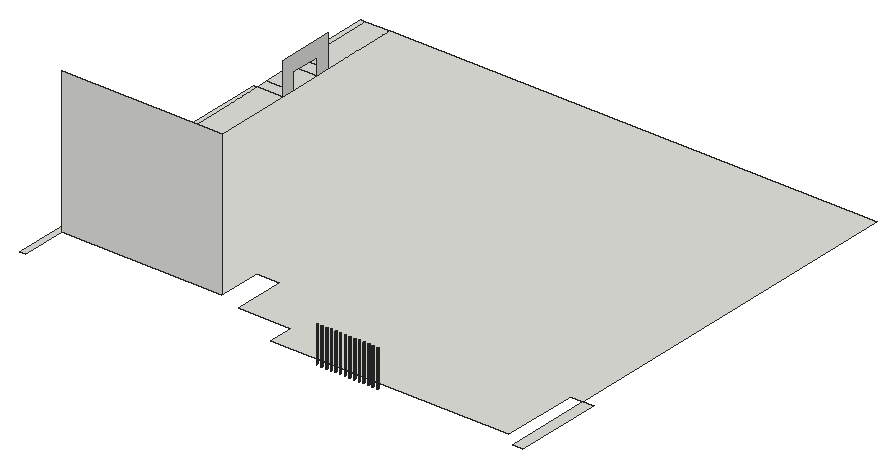
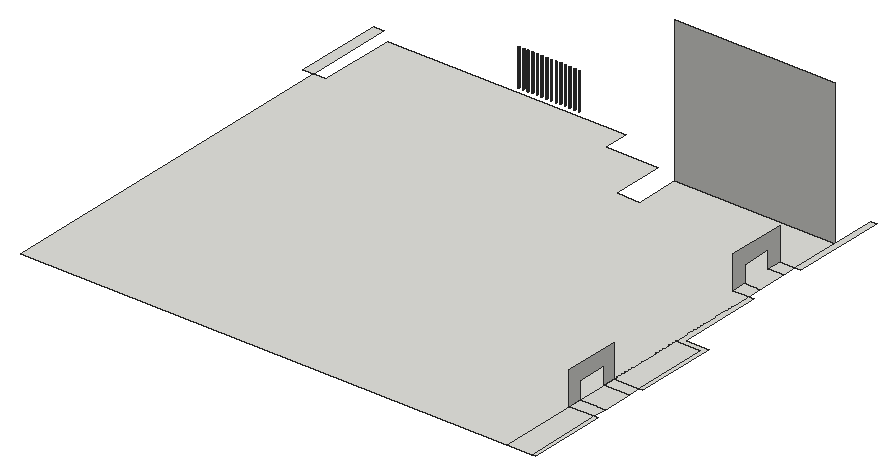
# SketchUp Ruby script. Lengths in inches.
U = 1.inch
M = Sketchup.active_model
def pt(a) = Geom::Point3d.new(a.map { |v| v * U })
def face(e, loops, mat)
  f = e.add_face(loops[0].map { |a| pt(a) })
  loops[1..].each { |l| e.add_face(l.map { |a| pt(a) }).erase! }
  f.material = f.back_material = mat if mat
  f
end
# faces: each face lists its corners as indices into pts; further lists are holes
def faces(e, pts, list, mat = nil) = list.each { |f| face(e, (f[0].is_a?(Array) ? f : [f]).map { |l| l.map { |i| pts[i] } }, mat) }
# xy, xz, yz: faces in a plane at the given z, y or x. An outline is a flat list of corners, or four numbers for a rectangle; further outlines are holes
def ring(l) = l.size == 4 ? [[l[0], l[1]], [l[2], l[1]], [l[2], l[3]], [l[0], l[3]]] : l.each_slice(2).to_a
def flat(e, list, mat, &to3) = list.each { |f| face(e, (f[0].is_a?(Array) ? f : [f]).map { |l| ring(l).map { |u, v| to3.(u, v) } }, mat) }
def xy(e, z, list, mat = nil) = flat(e, list, mat) { |x, y| [x, y, z] }
def xz(e, y, list, mat = nil) = flat(e, list, mat) { |x, z| [x, y, z] }
def yz(e, x, list, mat = nil) = flat(e, list, mat) { |y, z| [x, y, z] }
def lines(e, pts, list) = list.each { |a, b| e.add_line(pt(pts[a]), pt(pts[b])) }
# prism: a flat outline (further loops are holes) pulled along v
def prism(e, loops, v, mat = nil)
  f = face(e, loops, mat); d = Geom::Vector3d.new(v.map { |x| x * U })
  f.pushpull(f.normal.samedirection?(d) ? d.length : -d.length)
end
def box(e, o, s, mat = nil) = prism(e, [[o, [o[0] + s[0], o[1], o[2]], [o[0] + s[0], o[1] + s[1], o[2]], [o[0], o[1] + s[1], o[2]]]], [0, 0, s[2]], mat)
def at(x, y, z, deg = 0) = Geom::Transformation.translation(pt([x, y, z])) * Geom::Transformation.rotation(ORIGIN, Z_AXIS, deg.degrees)
def axes(o, x, y, z) = Geom::Transformation.new([*x, 0, *y, 0, *z, 0, *pt(o).to_a, 1])
def part(name) = M.definitions.add(name)
# library, detail: a bought-in or finely detailed component or shape, given as its bounding box
def library(name, o, s) = part(name).tap { |d| box(d.entities, o, s) }
def detail(e, o, s) = box(e.add_group.entities, o, s)
def put(e, d, t, mat = nil) = e.add_instance(d, t).tap { |i| i.material = mat if mat }
def group(e, t, mat = nil) = e.add_group.tap { |g| g.transformation = t; g.material = mat if mat }.entities
root = M.entities
M.materials.add("Generic\#2").color = [186, 186, 186]
xy(root,1024.6875,[[41,124.5,48.5,249],[690.4375,124.5,703.6875,241.25],[359.25,139.4375,673.48,139.4375,673.48,241.25,690.4375,241.25,690.4375,724.5,48.5,724.5,48.5,326.1875,69,326.1875,69,306.87,48.5,306.87,48.5,268.32,69,268.32,69,249,48.5,249,48.5,183.25,259.3125,183.25,259.3125,241.25,290.4375,241.25,290.4375,172.5,359.25,172.5],[48.5,249,69,268.32],[48.5,306.87,69,326.1875],
  [41,326.1875,48.5,326.1875,48.5,446.1875,15.3125,446.1875,15.3125,547.73,10.5,547.73,10.5,438.6875,41,438.6875],[15.3125,446.1875,48.5,547.73],[15.3125,547.73,48.5,563.94],[15.3125,563.94,48.5,603.53],[15.3125,603.53,48.5,621.86],
  [10.5,621.86,15.3125,724.5],[15.3125,621.86,48.5,724.5]])
xz(root,183.25,[[48.5,1024.6875,259.3125,1214.9375]])
yz(root,48.5,[[547.73,1024.6875,563.94,1024.6875,563.94,1046.8125,603.53,1046.8125,603.53,1024.6875,621.86,1024.6875,621.86,1067.5625,547.73,1067.5625]])
yz(root,69,[[249,1024.6875,268.32,1024.6875,268.32,1046.8125,306.87,1046.8125,306.87,1024.6875,326.1875,1024.6875,326.1875,1067.5625,249,1067.5625]])
p = [[427.76,129.86,1024.6875],[427.96,129.78,1024.6875],[427.96,129.78,1072.38],[427.76,129.86,1072.38],[428.17,129.75,1024.6875],[428.17,129.75,1072.38],
  [428.38,129.78,1024.6875],[428.38,129.78,1072.38],[428.57,129.86,1024.6875],[428.57,129.86,1072.38],[433.82,129.86,1024.6875],[434.02,129.78,1024.6875],
  [434.02,129.78,1072.38],[433.82,129.86,1072.38],[434.23,129.75,1024.6875],[434.23,129.75,1072.38],[434.44,129.78,1024.6875],[434.44,129.78,1072.38],
  [434.64,129.86,1024.6875],[434.64,129.86,1072.38],[439.95,129.86,1024.6875],[440.15,129.78,1024.6875],[440.15,129.78,1072.38],[439.95,129.86,1072.38],
  [440.36,129.75,1024.6875],[440.36,129.75,1072.38],[440.57,129.78,1024.6875],[440.57,129.78,1072.38],[440.76,129.86,1024.6875],[440.76,129.86,1072.38],
  [445.95,129.86,1024.6875],[446.15,129.78,1024.6875],[446.15,129.78,1072.38],[445.95,129.86,1072.38],[446.36,129.75,1024.6875],[446.36,129.75,1072.38],
  [446.57,129.78,1024.6875],[446.57,129.78,1072.38],[446.76,129.86,1024.6875],[446.76,129.86,1072.38],[452.2,129.86,1024.6875],[452.4,129.78,1024.6875],
  [452.4,129.78,1072.38],[452.2,129.86,1072.38],[452.61,129.75,1024.6875],[452.61,129.75,1072.38],[452.82,129.78,1024.6875],[452.82,129.78,1072.38],
  [453.01,129.86,1024.6875],[453.01,129.86,1072.38],[458.14,129.86,1024.6875],[458.33,129.78,1024.6875],[458.33,129.78,1072.38],[458.14,129.86,1072.38],
  [458.54,129.75,1024.6875],[458.54,129.75,1072.38],[458.75,129.78,1024.6875],[458.75,129.78,1072.38],[458.95,129.86,1024.6875],[458.95,129.86,1072.38],
  [464.39,129.86,1024.6875],[464.58,129.78,1024.6875],[464.58,129.78,1072.38],[464.39,129.86,1072.38],[464.79,129.75,1024.6875],[464.79,129.75,1072.38],
  [465,129.78,1024.6875],[465,129.78,1072.38],[465.2,129.86,1024.6875],[465.2,129.86,1072.38],[470.76,129.86,1024.6875],[470.96,129.78,1024.6875],
  [470.96,129.78,1072.38],[470.76,129.86,1072.38],[471.17,129.75,1024.6875],[471.17,129.75,1072.38],[471.38,129.78,1024.6875],[471.38,129.78,1072.38],
  [471.57,129.86,1024.6875],[471.57,129.86,1072.38],[476.76,129.86,1024.6875],[476.96,129.78,1024.6875],[476.96,129.78,1072.38],[476.76,129.86,1072.38],
  [477.17,129.75,1024.6875],[477.17,129.75,1072.38],[477.38,129.78,1024.6875],[477.38,129.78,1072.38],[477.57,129.86,1024.6875],[477.57,129.86,1072.38],
  [482.82,129.86,1024.6875],[483.02,129.78,1024.6875],[483.02,129.78,1072.38],[482.82,129.86,1072.38],[483.23,129.75,1024.6875],[483.23,129.75,1072.38],
  [483.44,129.78,1024.6875],[483.44,129.78,1072.38],[483.64,129.86,1024.6875],[483.64,129.86,1072.38],[489.2,129.86,1024.6875],[489.4,129.78,1024.6875],
  [489.4,129.78,1072.38],[489.2,129.86,1072.38],[489.61,129.75,1024.6875],[489.61,129.75,1072.38],[489.82,129.78,1024.6875],[489.82,129.78,1072.38],
  [490.01,129.86,1024.6875],[490.01,129.86,1072.38],[495.2,129.86,1024.6875],[495.4,129.78,1024.6875],[495.4,129.78,1072.38],[495.2,129.86,1072.38],
  [495.61,129.75,1024.6875],[495.61,129.75,1072.38],[495.82,129.78,1024.6875],[495.82,129.78,1072.38],[496.01,129.86,1024.6875],[496.01,129.86,1072.38],
  [501.2,129.86,1024.6875],[501.4,129.78,1024.6875],[501.4,129.78,1072.38],[501.2,129.86,1072.38],[501.61,129.75,1024.6875],[501.61,129.75,1072.38],
  [501.82,129.78,1024.6875],[501.82,129.78,1072.38],[502.01,129.86,1024.6875],[502.01,129.86,1072.38],[507.2,129.86,1024.6875],[507.4,129.78,1024.6875],
  [507.4,129.78,1072.38],[507.2,129.86,1072.38],[507.61,129.75,1024.6875],[507.61,129.75,1072.38],[507.82,129.78,1024.6875],[507.82,129.78,1072.38],
  [508.01,129.86,1024.6875],[508.01,129.86,1072.38],[427.59,129.99,1024.6875],[427.59,129.99,1072.38],[433.66,129.99,1024.6875],[433.66,129.99,1072.38],
  [434.81,129.99,1024.6875],[434.81,129.99,1072.38],[439.78,129.99,1024.6875],[439.78,129.99,1072.38],[440.93,129.99,1024.6875],[440.93,129.99,1072.38],
  [445.78,129.99,1024.6875],[445.78,129.99,1072.38],[446.93,129.99,1024.6875],[446.93,129.99,1072.38],[452.03,129.99,1024.6875],[452.03,129.99,1072.38],
  [453.18,129.99,1024.6875],[453.18,129.99,1072.38],[457.97,129.99,1024.6875],[457.97,129.99,1072.38],[459.12,129.99,1024.6875],[459.12,129.99,1072.38],
  [464.22,129.99,1024.6875],[464.22,129.99,1072.38],[465.37,129.99,1024.6875],[465.37,129.99,1072.38],[470.59,129.99,1024.6875],[470.59,129.99,1072.38],
  [471.74,129.99,1024.6875],[471.74,129.99,1072.38],[476.59,129.99,1024.6875],[476.59,129.99,1072.38],[477.74,129.99,1024.6875],[477.74,129.99,1072.38],
  [482.66,129.99,1024.6875],[482.66,129.99,1072.38],[483.81,129.99,1024.6875],[483.81,129.99,1072.38],[489.03,129.99,1024.6875],[489.03,129.99,1072.38],
  [490.18,129.99,1024.6875],[490.18,129.99,1072.38],[495.03,129.99,1024.6875],[495.03,129.99,1072.38],[496.18,129.99,1024.6875],[496.18,129.99,1072.38],
  [501.03,129.99,1024.6875],[501.03,129.99,1072.38],[502.18,129.99,1024.6875],[502.18,129.99,1072.38],[507.03,129.99,1024.6875],[507.03,129.99,1072.38],
  [508.18,129.99,1024.6875],[508.18,129.99,1072.38],[427.46,130.16,1024.6875],[427.46,130.16,1072.38],[433.53,130.16,1024.6875],[433.53,130.16,1072.38],
  [434.93,130.16,1024.6875],[434.93,130.16,1072.38],[439.65,130.16,1024.6875],[439.65,130.16,1072.38],[441.06,130.16,1024.6875],[441.06,130.16,1072.38],
  [445.65,130.16,1024.6875],[445.65,130.16,1072.38],[447.06,130.16,1024.6875],[447.06,130.16,1072.38],[451.9,130.16,1024.6875],[451.9,130.16,1072.38],
  [453.31,130.16,1024.6875],[453.31,130.16,1072.38],[457.84,130.16,1024.6875],[457.84,130.16,1072.38],[459.25,130.16,1024.6875],[459.25,130.16,1072.38],
  [464.09,130.16,1024.6875],[464.09,130.16,1072.38],[465.5,130.16,1024.6875],[465.5,130.16,1072.38],[470.46,130.16,1024.6875],[470.46,130.16,1072.38],
  [471.87,130.16,1024.6875],[471.87,130.16,1072.38],[476.46,130.16,1024.6875],[476.46,130.16,1072.38],[477.87,130.16,1024.6875],[477.87,130.16,1072.38],
  [482.53,130.16,1024.6875],[482.53,130.16,1072.38],[483.93,130.16,1024.6875],[483.93,130.16,1072.38],[488.9,130.16,1024.6875],[488.9,130.16,1072.38],
  [490.31,130.16,1024.6875],[490.31,130.16,1072.38],[494.9,130.16,1024.6875],[494.9,130.16,1072.38],[496.31,130.16,1024.6875],[496.31,130.16,1072.38],
  [500.9,130.16,1024.6875],[500.9,130.16,1072.38],[502.31,130.16,1024.6875],[502.31,130.16,1072.38],[506.9,130.16,1024.6875],[506.9,130.16,1072.38],
  [508.31,130.16,1024.6875],[508.31,130.16,1072.38],[427.38,130.36,1024.6875],[427.38,130.36,1072.38],[433.45,130.36,1024.6875],[433.45,130.36,1072.38],
  [435.02,130.36,1024.6875],[435.02,130.36,1072.38],[439.57,130.36,1024.6875],[439.57,130.36,1072.38],[441.14,130.36,1024.6875],[441.14,130.36,1072.38],
  [445.57,130.36,1024.6875],[445.57,130.36,1072.38],[447.14,130.36,1024.6875],[447.14,130.36,1072.38],[451.82,130.36,1024.6875],[451.82,130.36,1072.38],
  [453.39,130.36,1024.6875],[453.39,130.36,1072.38],[457.76,130.36,1024.6875],[457.76,130.36,1072.38],[459.33,130.36,1024.6875],[459.33,130.36,1072.38],
  [464.01,130.36,1024.6875],[464.01,130.36,1072.38],[465.58,130.36,1024.6875],[465.58,130.36,1072.38],[470.38,130.36,1024.6875],[470.38,130.36,1072.38],
  [471.95,130.36,1024.6875],[471.95,130.36,1072.38],[476.38,130.36,1024.6875],[476.38,130.36,1072.38],[477.95,130.36,1024.6875],[477.95,130.36,1072.38],
  [482.45,130.36,1024.6875],[482.45,130.36,1072.38],[484.02,130.36,1024.6875],[484.02,130.36,1072.38],[488.82,130.36,1024.6875],[488.82,130.36,1072.38],
  [490.39,130.36,1024.6875],[490.39,130.36,1072.38],[494.82,130.36,1024.6875],[494.82,130.36,1072.38],[496.39,130.36,1024.6875],[496.39,130.36,1072.38],
  [500.82,130.36,1024.6875],[500.82,130.36,1072.38],[502.39,130.36,1024.6875],[502.39,130.36,1072.38],[506.82,130.36,1024.6875],[506.82,130.36,1072.38],
  [508.39,130.36,1024.6875],[508.39,130.36,1072.38],[427.36,130.57,1024.6875],[427.36,130.57,1072.38],[433.42,130.57,1024.6875],[433.42,130.57,1072.38],
  [435.04,130.57,1024.6875],[435.04,130.57,1072.38],[439.54,130.57,1024.6875],[439.54,130.57,1072.38],[441.17,130.57,1024.6875],[441.17,130.57,1072.38],
  [445.54,130.57,1024.6875],[445.54,130.57,1072.38],[447.17,130.57,1024.6875],[447.17,130.57,1072.38],[451.79,130.57,1024.6875],[451.79,130.57,1072.38],
  [453.42,130.57,1024.6875],[453.42,130.57,1072.38],[457.73,130.57,1024.6875],[457.73,130.57,1072.38],[459.36,130.57,1024.6875],[459.36,130.57,1072.38],
  [463.98,130.57,1024.6875],[463.98,130.57,1072.38],[465.61,130.57,1024.6875],[465.61,130.57,1072.38],[470.36,130.57,1024.6875],[470.36,130.57,1072.38],
  [471.98,130.57,1024.6875],[471.98,130.57,1072.38],[476.36,130.57,1024.6875],[476.36,130.57,1072.38],[477.98,130.57,1024.6875],[477.98,130.57,1072.38],
  [482.42,130.57,1024.6875],[482.42,130.57,1072.38],[484.04,130.57,1024.6875],[484.04,130.57,1072.38],[488.79,130.57,1024.6875],[488.79,130.57,1072.38],
  [490.42,130.57,1024.6875],[490.42,130.57,1072.38],[494.79,130.57,1024.6875],[494.79,130.57,1072.38],[496.42,130.57,1024.6875],[496.42,130.57,1072.38],
  [500.79,130.57,1024.6875],[500.79,130.57,1072.38],[502.42,130.57,1024.6875],[502.42,130.57,1072.38],[506.79,130.57,1024.6875],[506.79,130.57,1072.38],
  [508.42,130.57,1024.6875],[508.42,130.57,1072.38],[427.38,130.78,1024.6875],[427.38,130.78,1072.38],[433.45,130.78,1024.6875],[433.45,130.78,1072.38],
  [435.02,130.78,1024.6875],[435.02,130.78,1072.38],[439.57,130.78,1024.6875],[439.57,130.78,1072.38],[441.14,130.78,1024.6875],[441.14,130.78,1072.38],
  [445.57,130.78,1024.6875],[445.57,130.78,1072.38],[447.14,130.78,1024.6875],[447.14,130.78,1072.38],[451.82,130.78,1024.6875],[451.82,130.78,1072.38],
  [453.39,130.78,1024.6875],[453.39,130.78,1072.38],[457.76,130.78,1024.6875],[457.76,130.78,1072.38],[459.33,130.78,1024.6875],[459.33,130.78,1072.38],
  [464.01,130.78,1024.6875],[464.01,130.78,1072.38],[465.58,130.78,1024.6875],[465.58,130.78,1072.38],[470.38,130.78,1024.6875],[470.38,130.78,1072.38],
  [471.95,130.78,1024.6875],[471.95,130.78,1072.38],[476.38,130.78,1024.6875],[476.38,130.78,1072.38],[477.95,130.78,1024.6875],[477.95,130.78,1072.38],
  [482.45,130.78,1024.6875],[482.45,130.78,1072.38],[484.02,130.78,1024.6875],[484.02,130.78,1072.38],[488.82,130.78,1024.6875],[488.82,130.78,1072.38],
  [490.39,130.78,1024.6875],[490.39,130.78,1072.38],[494.82,130.78,1024.6875],[494.82,130.78,1072.38],[496.39,130.78,1024.6875],[496.39,130.78,1072.38],
  [500.82,130.78,1024.6875],[500.82,130.78,1072.38],[502.39,130.78,1024.6875],[502.39,130.78,1072.38],[506.82,130.78,1024.6875],[506.82,130.78,1072.38],
  [508.39,130.78,1024.6875],[508.39,130.78,1072.38],[427.46,130.97,1024.6875],[427.46,130.97,1072.38],[433.53,130.97,1024.6875],[433.53,130.97,1072.38],
  [434.93,130.97,1024.6875],[434.93,130.97,1072.38],[439.65,130.97,1024.6875],[439.65,130.97,1072.38],[441.06,130.97,1024.6875],[441.06,130.97,1072.38],
  [445.65,130.97,1024.6875],[445.65,130.97,1072.38],[447.06,130.97,1024.6875],[447.06,130.97,1072.38],[451.9,130.97,1024.6875],[451.9,130.97,1072.38],
  [453.31,130.97,1024.6875],[453.31,130.97,1072.38],[457.84,130.97,1024.6875],[457.84,130.97,1072.38],[459.25,130.97,1024.6875],[459.25,130.97,1072.38],
  [464.09,130.97,1024.6875],[464.09,130.97,1072.38],[465.5,130.97,1024.6875],[465.5,130.97,1072.38],[470.46,130.97,1024.6875],[470.46,130.97,1072.38],
  [471.87,130.97,1024.6875],[471.87,130.97,1072.38],[476.46,130.97,1024.6875],[476.46,130.97,1072.38],[477.87,130.97,1024.6875],[477.87,130.97,1072.38],
  [482.53,130.97,1024.6875],[482.53,130.97,1072.38],[483.93,130.97,1024.6875],[483.93,130.97,1072.38],[488.9,130.97,1024.6875],[488.9,130.97,1072.38],
  [490.31,130.97,1024.6875],[490.31,130.97,1072.38],[494.9,130.97,1024.6875],[494.9,130.97,1072.38],[496.31,130.97,1024.6875],[496.31,130.97,1072.38],
  [500.9,130.97,1024.6875],[500.9,130.97,1072.38],[502.31,130.97,1024.6875],[502.31,130.97,1072.38],[506.9,130.97,1024.6875],[506.9,130.97,1072.38],
  [508.31,130.97,1024.6875],[508.31,130.97,1072.38],[427.59,131.14,1024.6875],[427.59,131.14,1072.38],[433.66,131.14,1024.6875],[433.66,131.14,1072.38],
  [434.81,131.14,1024.6875],[434.81,131.14,1072.38],[439.78,131.14,1024.6875],[439.78,131.14,1072.38],[440.93,131.14,1024.6875],[440.93,131.14,1072.38],
  [445.78,131.14,1024.6875],[445.78,131.14,1072.38],[446.93,131.14,1024.6875],[446.93,131.14,1072.38],[452.03,131.14,1024.6875],[452.03,131.14,1072.38],
  [453.18,131.14,1024.6875],[453.18,131.14,1072.38],[457.97,131.14,1024.6875],[457.97,131.14,1072.38],[459.12,131.14,1024.6875],[459.12,131.14,1072.38],
  [464.22,131.14,1024.6875],[464.22,131.14,1072.38],[465.37,131.14,1024.6875],[465.37,131.14,1072.38],[470.59,131.14,1024.6875],[470.59,131.14,1072.38],
  [471.74,131.14,1024.6875],[471.74,131.14,1072.38],[476.59,131.14,1024.6875],[476.59,131.14,1072.38],[477.74,131.14,1024.6875],[477.74,131.14,1072.38],
  [482.66,131.14,1024.6875],[482.66,131.14,1072.38],[483.81,131.14,1024.6875],[483.81,131.14,1072.38],[489.03,131.14,1024.6875],[489.03,131.14,1072.38],
  [490.18,131.14,1024.6875],[490.18,131.14,1072.38],[495.03,131.14,1024.6875],[495.03,131.14,1072.38],[496.18,131.14,1024.6875],[496.18,131.14,1072.38],
  [501.03,131.14,1024.6875],[501.03,131.14,1072.38],[502.18,131.14,1024.6875],[502.18,131.14,1072.38],[507.03,131.14,1024.6875],[507.03,131.14,1072.38],
  [508.18,131.14,1024.6875],[508.18,131.14,1072.38],[433.82,131.27,1024.6875],[433.82,131.27,1072.38],[434.64,131.27,1024.6875],[434.64,131.27,1072.38],
  [439.95,131.27,1024.6875],[439.95,131.27,1072.38],[440.76,131.27,1024.6875],[440.76,131.27,1072.38],[445.95,131.27,1024.6875],[445.95,131.27,1072.38],
  [446.76,131.27,1024.6875],[446.76,131.27,1072.38],[452.2,131.27,1024.6875],[452.2,131.27,1072.38],[453.01,131.27,1024.6875],[453.01,131.27,1072.38],
  [458.14,131.27,1024.6875],[458.14,131.27,1072.38],[458.95,131.27,1024.6875],[458.95,131.27,1072.38],[464.39,131.27,1024.6875],[464.39,131.27,1072.38],
  [465.2,131.27,1024.6875],[465.2,131.27,1072.38],[470.76,131.27,1024.6875],[470.76,131.27,1072.38],[471.57,131.27,1024.6875],[471.57,131.27,1072.38],
  [476.76,131.27,1024.6875],[476.76,131.27,1072.38],[477.57,131.27,1024.6875],[477.57,131.27,1072.38],[482.82,131.27,1024.6875],[482.82,131.27,1072.38],
  [483.64,131.27,1024.6875],[483.64,131.27,1072.38],[489.2,131.27,1024.6875],[489.2,131.27,1072.38],[490.01,131.27,1024.6875],[490.01,131.27,1072.38],
  [495.2,131.27,1024.6875],[495.2,131.27,1072.38],[496.01,131.27,1024.6875],[496.01,131.27,1072.38],[501.2,131.27,1024.6875],[501.2,131.27,1072.38],
  [502.01,131.27,1024.6875],[502.01,131.27,1072.38],[507.2,131.27,1024.6875],[507.2,131.27,1072.38],[508.01,131.27,1024.6875],[508.01,131.27,1072.38],
  [434.02,131.35,1024.6875],[434.02,131.35,1072.38],[434.44,131.35,1024.6875],[434.44,131.35,1072.38],[440.15,131.35,1024.6875],[440.15,131.35,1072.38],
  [440.57,131.35,1024.6875],[440.57,131.35,1072.38],[446.15,131.35,1024.6875],[446.15,131.35,1072.38],[446.57,131.35,1024.6875],[446.57,131.35,1072.38],
  [452.4,131.35,1024.6875],[452.4,131.35,1072.38],[452.82,131.35,1024.6875],[452.82,131.35,1072.38],[458.33,131.35,1024.6875],[458.33,131.35,1072.38],
  [458.75,131.35,1024.6875],[458.75,131.35,1072.38],[464.58,131.35,1024.6875],[464.58,131.35,1072.38],[465,131.35,1024.6875],[465,131.35,1072.38],
  [470.96,131.35,1024.6875],[470.96,131.35,1072.38],[471.38,131.35,1024.6875],[471.38,131.35,1072.38],[476.96,131.35,1024.6875],[476.96,131.35,1072.38],
  [477.38,131.35,1024.6875],[477.38,131.35,1072.38],[483.02,131.35,1024.6875],[483.02,131.35,1072.38],[483.44,131.35,1024.6875],[483.44,131.35,1072.38],
  [489.4,131.35,1024.6875],[489.4,131.35,1072.38],[489.82,131.35,1024.6875],[489.82,131.35,1072.38],[495.4,131.35,1024.6875],[495.4,131.35,1072.38],
  [495.82,131.35,1024.6875],[495.82,131.35,1072.38],[501.4,131.35,1024.6875],[501.4,131.35,1072.38],[501.82,131.35,1024.6875],[501.82,131.35,1072.38],
  [507.4,131.35,1024.6875],[507.4,131.35,1072.38],[507.82,131.35,1024.6875],[507.82,131.35,1072.38],[434.23,131.38,1024.6875],[434.23,131.38,1072.38],
  [440.36,131.38,1024.6875],[440.36,131.38,1072.38],[446.36,131.38,1024.6875],[446.36,131.38,1072.38],[452.61,131.38,1024.6875],[452.61,131.38,1072.38],
  [458.54,131.38,1024.6875],[458.54,131.38,1072.38],[464.79,131.38,1024.6875],[464.79,131.38,1072.38],[471.17,131.38,1024.6875],[471.17,131.38,1072.38],
  [477.17,131.38,1024.6875],[477.17,131.38,1072.38],[483.23,131.38,1024.6875],[483.23,131.38,1072.38],[489.61,131.38,1024.6875],[489.61,131.38,1072.38],
  [495.61,131.38,1024.6875],[495.61,131.38,1072.38],[501.61,131.38,1024.6875],[501.61,131.38,1072.38],[507.61,131.38,1024.6875],[507.61,131.38,1072.38]]
faces(root,p,[[0,1,2,3],[1,4,5,2],[4,6,7,5],[6,8,9,7],[10,11,12,13],[11,14,15,12],[14,16,17,15],[16,18,19,17],
  [20,21,22,23],[21,24,25,22],[24,26,27,25],[26,28,29,27],[30,31,32,33],[31,34,35,32],[34,36,37,35],[36,38,39,37],
  [40,41,42,43],[41,44,45,42],[44,46,47,45],[46,48,49,47],[50,51,52,53],[51,54,55,52],[54,56,57,55],[56,58,59,57],
  [60,61,62,63],[61,64,65,62],[64,66,67,65],[66,68,69,67],[70,71,72,73],[71,74,75,72],[74,76,77,75],[76,78,79,77],
  [80,81,82,83],[81,84,85,82],[84,86,87,85],[86,88,89,87],[90,91,92,93],[91,94,95,92],[94,96,97,95],[96,98,99,97],
  [100,101,102,103],[101,104,105,102],[104,106,107,105],[106,108,109,107],[110,111,112,113],[111,114,115,112],[114,116,117,115],[116,118,119,117],
  [120,121,122,123],[121,124,125,122],[124,126,127,125],[126,128,129,127],[130,131,132,133],[131,134,135,132],[134,136,137,135],[136,138,139,137],
  [140,0,3,141],[142,10,13,143],[18,144,145,19],[146,20,23,147],[28,148,149,29],[150,30,33,151],[38,152,153,39],[154,40,43,155],
  [48,156,157,49],[158,50,53,159],[58,160,161,59],[162,60,63,163],[68,164,165,69],[166,70,73,167],[78,168,169,79],[170,80,83,171],
  [88,172,173,89],[174,90,93,175],[98,176,177,99],[178,100,103,179],[108,180,181,109],[182,110,113,183],[118,184,185,119],[186,120,123,187],
  [128,188,189,129],[190,130,133,191],[138,192,193,139],[194,140,141,195],[196,142,143,197],[144,198,199,145],[200,146,147,201],[148,202,203,149],
  [204,150,151,205],[152,206,207,153],[208,154,155,209],[156,210,211,157],[212,158,159,213],[160,214,215,161],[216,162,163,217],[164,218,219,165],
  [220,166,167,221],[168,222,223,169],[224,170,171,225],[172,226,227,173],[228,174,175,229],[176,230,231,177],[232,178,179,233],[180,234,235,181],
  [236,182,183,237],[184,238,239,185],[240,186,187,241],[188,242,243,189],[244,190,191,245],[192,246,247,193],[248,194,195,249],[250,196,197,251],
  [198,252,253,199],[254,200,201,255],[202,256,257,203],[258,204,205,259],[206,260,261,207],[262,208,209,263],[210,264,265,211],[266,212,213,267],
  [214,268,269,215],[270,216,217,271],[218,272,273,219],[274,220,221,275],[222,276,277,223],[278,224,225,279],[226,280,281,227],[282,228,229,283],
  [230,284,285,231],[286,232,233,287],[234,288,289,235],[290,236,237,291],[238,292,293,239],[294,240,241,295],[242,296,297,243],[298,244,245,299],
  [246,300,301,247],[302,248,249,303],[304,250,251,305],[252,306,307,253],[308,254,255,309],[256,310,311,257],[312,258,259,313],[260,314,315,261],
  [316,262,263,317],[264,318,319,265],[320,266,267,321],[268,322,323,269],[324,270,271,325],[272,326,327,273],[328,274,275,329],[276,330,331,277],
  [332,278,279,333],[280,334,335,281],[336,282,283,337],[284,338,339,285],[340,286,287,341],[288,342,343,289],[344,290,291,345],[292,346,347,293],
  [348,294,295,349],[296,350,351,297],[352,298,299,353],[300,354,355,301],[356,302,303,357],[358,304,305,359],[306,360,361,307],[362,308,309,363],
  [310,364,365,311],[366,312,313,367],[314,368,369,315],[370,316,317,371],[318,372,373,319],[374,320,321,375],[322,376,377,323],[378,324,325,379],
  [326,380,381,327],[382,328,329,383],[330,384,385,331],[386,332,333,387],[334,388,389,335],[390,336,337,391],[338,392,393,339],[394,340,341,395],
  [342,396,397,343],[398,344,345,399],[346,400,401,347],[402,348,349,403],[350,404,405,351],[406,352,353,407],[354,408,409,355],[410,356,357,411],
  [412,358,359,413],[360,414,415,361],[416,362,363,417],[364,418,419,365],[420,366,367,421],[368,422,423,369],[424,370,371,425],[372,426,427,373],
  [428,374,375,429],[376,430,431,377],[432,378,379,433],[380,434,435,381],[436,382,383,437],[384,438,439,385],[440,386,387,441],[388,442,443,389],
  [444,390,391,445],[392,446,447,393],[448,394,395,449],[396,450,451,397],[452,398,399,453],[400,454,455,401],[456,402,403,457],[404,458,459,405],
  [460,406,407,461],[408,462,463,409],[464,410,411,465],[466,412,413,467],[414,468,469,415],[470,416,417,471],[418,472,473,419],[474,420,421,475],
  [422,476,477,423],[478,424,425,479],[426,480,481,427],[482,428,429,483],[430,484,485,431],[486,432,433,487],[434,488,489,435],[490,436,437,491],
  [438,492,493,439],[494,440,441,495],[442,496,497,443],[498,444,445,499],[446,500,501,447],[502,448,449,503],[450,504,505,451],[506,452,453,507],
  [454,508,509,455],[510,456,457,511],[458,512,513,459],[514,460,461,515],[462,516,517,463],[518,466,467,519],[468,520,521,469],[522,470,471,523],
  [472,524,525,473],[526,474,475,527],[476,528,529,477],[530,478,479,531],[480,532,533,481],[534,482,483,535],[484,536,537,485],[538,486,487,539],
  [488,540,541,489],[542,490,491,543],[492,544,545,493],[546,494,495,547],[496,548,549,497],[550,498,499,551],[500,552,553,501],[554,502,503,555],
  [504,556,557,505],[558,506,507,559],[508,560,561,509],[562,510,511,563],[512,564,565,513],[566,514,515,567],[516,568,569,517],[570,518,519,571],
  [520,572,573,521],[574,522,523,575],[524,576,577,525],[578,526,527,579],[528,580,581,529],[582,530,531,583],[532,584,585,533],[586,534,535,587],
  [536,588,589,537],[590,538,539,591],[540,592,593,541],[594,542,543,595],[544,596,597,545],[598,546,547,599],[548,600,601,549],[602,550,551,603],
  [552,604,605,553],[606,554,555,607],[556,608,609,557],[610,558,559,611],[560,612,613,561],[614,562,563,615],[564,616,617,565],[618,566,567,619],
  [568,620,621,569],[622,570,571,623],[572,622,623,573],[624,574,575,625],[576,624,625,577],[626,578,579,627],[580,626,627,581],[628,582,583,629],
  [584,628,629,585],[630,586,587,631],[588,630,631,589],[632,590,591,633],[592,632,633,593],[634,594,595,635],[596,634,635,597],[636,598,599,637],
  [600,636,637,601],[638,602,603,639],[604,638,639,605],[640,606,607,641],[608,640,641,609],[642,610,611,643],[612,642,643,613],[644,614,615,645],
  [616,644,645,617],[646,618,619,647],[620,646,647,621]],"Generic\#2")
